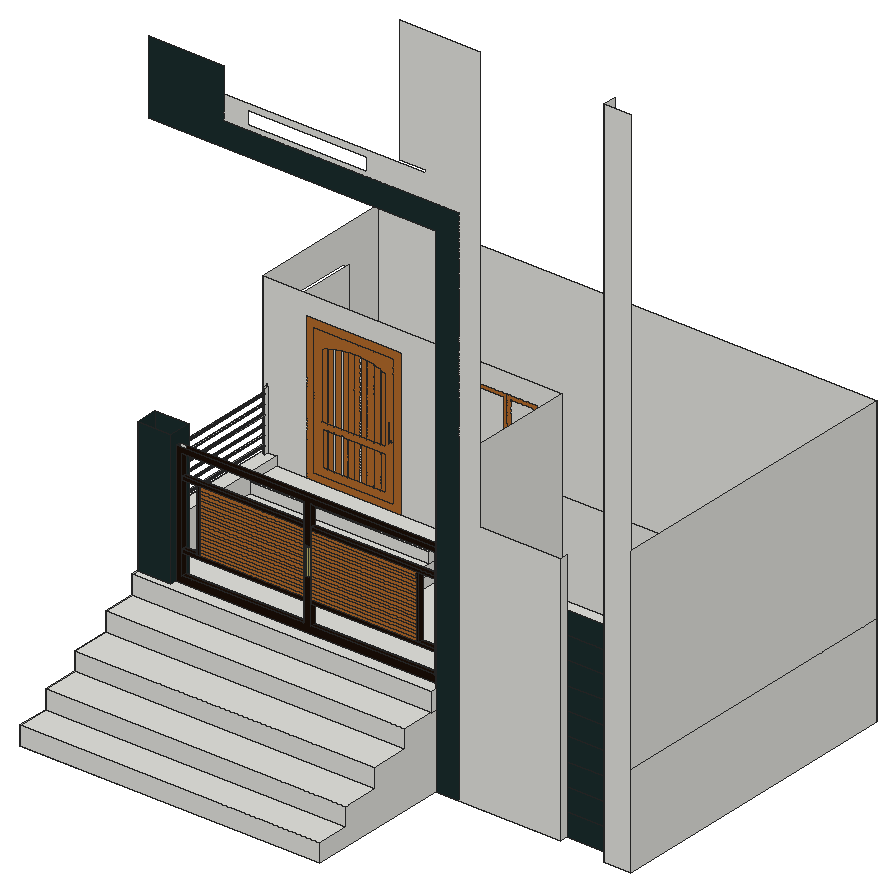
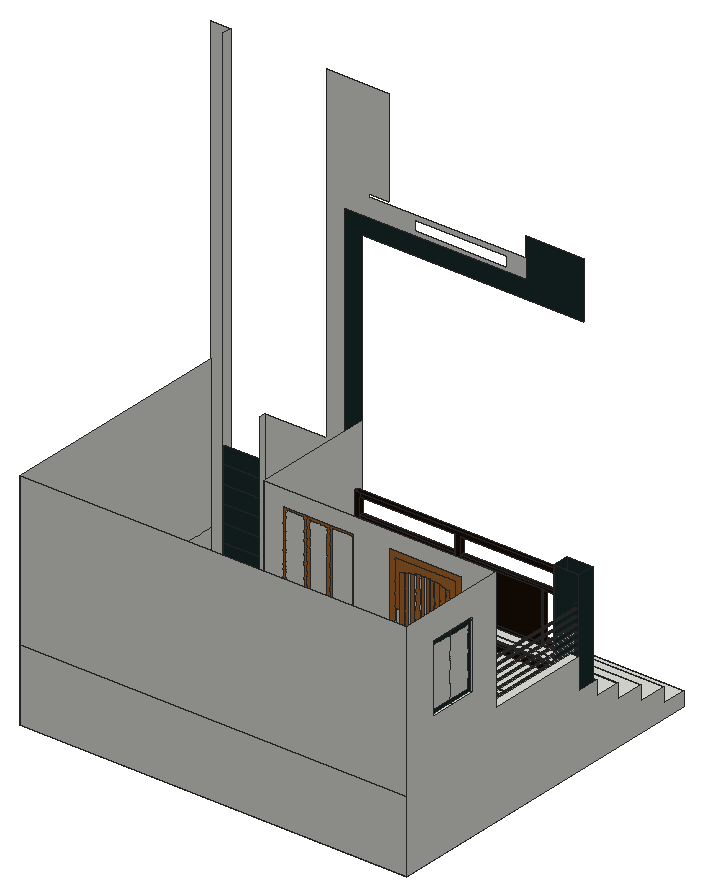
# SketchUp Ruby script. Lengths in inches.
U = 1.inch
M = Sketchup.active_model
def pt(a) = Geom::Point3d.new(a.map { |v| v * U })
def face(e, loops, mat)
  f = e.add_face(loops[0].map { |a| pt(a) })
  loops[1..].each { |l| e.add_face(l.map { |a| pt(a) }).erase! }
  f.material = f.back_material = mat if mat
  f
end
# faces: each face lists its corners as indices into pts; further lists are holes
def faces(e, pts, list, mat = nil) = list.each { |f| face(e, (f[0].is_a?(Array) ? f : [f]).map { |l| l.map { |i| pts[i] } }, mat) }
# xy, xz, yz: faces in a plane at the given z, y or x. An outline is a flat list of corners, or four numbers for a rectangle; further outlines are holes
def ring(l) = l.size == 4 ? [[l[0], l[1]], [l[2], l[1]], [l[2], l[3]], [l[0], l[3]]] : l.each_slice(2).to_a
def flat(e, list, mat, &to3) = list.each { |f| face(e, (f[0].is_a?(Array) ? f : [f]).map { |l| ring(l).map { |u, v| to3.(u, v) } }, mat) }
def xy(e, z, list, mat = nil) = flat(e, list, mat) { |x, y| [x, y, z] }
def xz(e, y, list, mat = nil) = flat(e, list, mat) { |x, z| [x, y, z] }
def yz(e, x, list, mat = nil) = flat(e, list, mat) { |y, z| [x, y, z] }
def lines(e, pts, list) = list.each { |a, b| e.add_line(pt(pts[a]), pt(pts[b])) }
# prism: a flat outline (further loops are holes) pulled along v
def prism(e, loops, v, mat = nil)
  f = face(e, loops, mat); d = Geom::Vector3d.new(v.map { |x| x * U })
  f.pushpull(f.normal.samedirection?(d) ? d.length : -d.length)
end
def box(e, o, s, mat = nil) = prism(e, [[o, [o[0] + s[0], o[1], o[2]], [o[0] + s[0], o[1] + s[1], o[2]], [o[0], o[1] + s[1], o[2]]]], [0, 0, s[2]], mat)
def at(x, y, z, deg = 0) = Geom::Transformation.translation(pt([x, y, z])) * Geom::Transformation.rotation(ORIGIN, Z_AXIS, deg.degrees)
def axes(o, x, y, z) = Geom::Transformation.new([*x, 0, *y, 0, *z, 0, *pt(o).to_a, 1])
def part(name) = M.definitions.add(name)
# library, detail: a bought-in or finely detailed component or shape, given as its bounding box
def library(name, o, s) = part(name).tap { |d| box(d.entities, o, s) }
def detail(e, o, s) = box(e.add_group.entities, o, s)
def put(e, d, t, mat = nil) = e.add_instance(d, t).tap { |i| i.material = mat if mat }
def group(e, t, mat = nil) = e.add_group.tap { |g| g.transformation = t; g.material = mat if mat }.entities
root = M.entities
M.materials.add("[0057_DarkKhaki]").color = [189, 183, 107]
M.materials.add("[0078_DarkSlateGray]").color = [27, 45, 45]
M.materials.add("[Wood Bamboo]").color = [177, 105, 43]
M.materials.add("[Wood Veneer 01]").color = [28, 16, 8]
xy(root,-50.5,[[13.625,0,13.625,274.0625,319.25,274.0625,319.25,85.75,303.01,85.75,303.01,93.625,273.68,93.625,273.68,88.9375,197.375,88.9375,197.375,0]])
xy(root,-39.2,[[13.625,0,197.375,19.5]])
xy(root,-27.9,[[13.625,19.5,197.375,42.0625]])
xy(root,-16.6,[[13.625,42.0625,197.375,65.25]])
xy(root,-5.3,[[13.625,65.25,197.375,85.75]])
xy(root,6,[[13.625,85.75,197.375,85.75,197.375,93.625,33.97,93.625,33.97,89.97,13.625,89.97],[33.97,96.69,197.375,96.69,197.375,185.5625,131.83,185.5625,131.83,141.5,22.27,141.5,22.27,103.41,33.97,103.41]])
xy(root,10.3125,[[37.47,93.625,112.35,96.69],[116.92,93.625,192.625,96.69]],"[Wood Veneer 01]")
xy(root,12.23,[[22.27,141.5,131.83,154.3125]])
xy(root,18.47,[[22.27,154.3125,131.83,165.4375]])
xy(root,22.63,[[37.47,93.625,112.35,96.69],[116.92,93.625,192.625,96.69]],"[Wood Veneer 01]")
xy(root,24.7,[[22.27,165.4375,131.83,185.5625]])
xy(root,24.71,[[46.66,93.625,48.59,96.69],[48.59,93.625,112.35,96.69],[116.92,93.625,181.16,96.69],[181.16,93.625,183.09,96.69]])
xy(root,24.71,[[37.47,93.625,46.66,96.69],[183.09,93.625,192.625,96.69]],"[Wood Veneer 01]")
xy(root,30.25,[[13.625,103.41,22.27,103.41,22.27,185.5625,17.09,185.5625,17.09,183.375,15.47,183.375,15.47,185.5625,13.625,185.5625]])
xy(root,37.79,[[113.13,92.625,114.51,93.625],[114.82,92.625,116.19,93.625]],"[0057_DarkKhaki]")
xy(root,45.65,[[16.23,103.41,16.39,183.375]])
xy(root,51.33,[[13.625,208.27,15.875,228.36],[15.875,208.27,16.1875,228.36],[13.625,228.36,15.875,248.45],[15.875,228.36,16.1875,248.45]])
xy(root,52.6,[[16.17,103.41,16.34,183.375]])
xy(root,53.42,[[113.13,92.625,114.51,93.625],[114.82,92.625,116.19,93.625]],"[0057_DarkKhaki]")
xy(root,62.69,[[46.66,93.625,48.59,96.69],[48.59,93.625,112.35,96.69],[116.92,93.625,181.16,96.69],[181.16,93.625,183.09,96.69]])
xy(root,62.69,[[37.47,93.625,46.66,96.69],[183.09,93.625,192.625,96.69]],"[Wood Veneer 01]")
xy(root,64.78,[[37.47,93.625,112.35,96.69],[116.92,93.625,192.625,96.69]],"[Wood Veneer 01]")
xz(root,0,[[13.625,-50.5,197.375,-39.2]])
xz(root,19.5,[[13.625,-39.2,197.375,-27.9]])
xz(root,42.0625,[[13.625,-27.9,197.375,-16.6]])
xz(root,65.25,[[13.625,-16.6,197.375,-5.3]])
xz(root,85.75,[[303.01,-50.5,319.25,365.8125],[13.625,-5.3,197.375,6]])
xz(root,88.9375,[[[211.43,-50.5,273.68,-50.5,273.68,104.5,224.51,104.5,224.51,365.8125,175.33,365.8125,175.33,289.25,191.33,289.25,191.33,287.4375,67.43,287.4375,67.43,272.375,211.43,272.375],[81.97,275.45,155.1,283.82]]])
xz(root,88.9375,[[197.375,-50.5,211.43,-50.5,211.43,272.375,67.43,272.375,67.43,302.875,21.25,302.875,21.25,258,197.375,258]],"[0078_DarkSlateGray]")
xz(root,89.97,[[13.625,6,33.97,88.125]],"[0078_DarkSlateGray]")
xz(root,92.625,[[113.13,37.79,114.51,53.42],[114.82,37.79,116.19,53.42]],"[0057_DarkKhaki]")
xz(root,93.625,[[273.68,-50.5,303.01,-36.62],[273.68,-36.62,303.01,-22.75],[273.68,-22.75,303.01,-8.87],[273.68,-8.87,303.01,5.01],[273.68,5.01,303.01,18.89],
  [273.68,18.89,303.01,32.76],[273.68,32.76,303.01,46.64],[273.68,46.64,303.01,60.52],[273.68,60.52,303.01,74.39]],"[0078_DarkSlateGray]")
xz(root,93.625,[[48.59,24.71,112.35,26.61],[116.92,24.71,181.16,26.61],[48.59,26.61,112.35,28.51],[116.92,26.61,181.16,28.51],[48.59,28.51,112.35,30.41],
  [116.92,28.51,181.16,30.41],[48.59,30.41,112.35,32.31],[116.92,30.41,181.16,32.31],[48.59,32.31,112.35,34.21],[116.92,32.31,181.16,34.21],
  [48.59,34.21,112.35,36.11],[116.92,34.21,181.16,36.11],[48.59,36.11,112.35,38.01],[116.92,36.11,181.16,38.01],[48.59,38.01,112.35,39.9],
  [116.92,38.01,181.16,39.9],[48.59,39.9,112.35,41.8],[116.92,39.9,181.16,41.8],[48.59,41.8,112.35,43.7],[116.92,41.8,181.16,43.7],
  [48.59,43.7,112.35,45.6],[116.92,43.7,181.16,45.6],[48.59,45.6,112.35,47.5],[116.92,45.6,181.16,47.5],[48.59,47.5,112.35,49.4],
  [116.92,47.5,181.16,49.4],[48.59,49.4,112.35,51.3],[116.92,49.4,181.16,51.3],[48.59,51.3,112.35,53.2],[116.92,51.3,181.16,53.2],
  [48.59,53.2,112.35,55.1],[116.92,53.2,181.16,55.1],[48.59,55.1,112.35,56.99],[116.92,55.1,181.16,56.99],[48.59,56.99,112.35,58.89],
  [116.92,56.99,181.16,58.89],[48.59,58.89,112.35,60.79],[116.92,58.89,181.16,60.79],[48.59,60.79,112.35,62.69],[116.92,60.79,181.16,62.69]],"[Wood Bamboo]")
xz(root,93.625,[[[33.97,6,197.375,80.73],[116.92,10.3125,192.625,77.61],[37.47,10.3125,112.35,77.61],[113.13,37.79,114.51,53.42],[114.82,37.79,116.19,53.42]],[37.47,22.63,112.35,24.71],[116.92,22.63,192.625,24.71],[46.66,24.71,48.59,62.69],[181.16,24.71,183.09,62.69],
  [37.47,62.69,112.35,64.78],[116.92,62.69,192.625,64.78]],"[Wood Veneer 01]")
xz(root,96.69,[[33.97,6,37.47,80.73]])
xz(root,96.69,[[37.47,6,192.625,10.3125],[192.625,6,197.375,80.73],[112.35,10.3125,116.92,24.71],[37.47,22.63,112.35,24.71],[116.92,22.63,192.625,24.71],
  [46.66,24.71,48.59,62.69],[48.59,24.71,112.35,62.69],[112.35,24.71,116.92,62.69],[116.92,24.71,181.16,62.69],[181.16,24.71,183.09,62.69],
  [112.35,62.69,112.35,77.61,37.47,77.61,37.47,80.73,192.625,80.73,192.625,77.61,116.92,77.61,116.92,62.69],[37.47,62.69,112.35,64.78],[116.92,62.69,192.625,64.78]],"[Wood Veneer 01]")
xz(root,103.41,[[[22.27,6,22.27,30.25,13.625,30.25,13.625,88.125,33.97,88.125,33.97,6],[15.47,66.44,17.09,68.06],[16.23,62.78,16.39,62.79,16.55,62.84,16.68,62.93,16.79,63.05,16.87,63.19,16.9,63.35,16.9,63.52,16.85,63.67,16.76,63.81,16.64,63.92,16.49,63.99,16.34,64.03,16.17,64.02,16.02,63.97,15.88,63.88,15.77,63.76,15.69,63.62,15.66,63.46,15.67,63.3,15.72,63.14,15.8,63,15.92,62.89,16.07,62.82],[16.23,57.07,16.39,57.08,16.55,57.13,16.68,57.22,16.79,57.34,16.87,57.48,16.9,57.64,16.9,57.8,16.85,57.96,16.76,58.1,16.64,58.21,16.49,58.28,16.34,58.32,16.17,58.31,16.02,58.26,15.88,58.17,15.77,58.05,15.69,57.91,15.66,57.75,15.67,57.58,15.72,57.43,15.8,57.29,15.92,57.18,16.07,57.11],[16.23,51.36,16.39,51.37,16.55,51.42,16.68,51.5,16.79,51.625,16.87,51.77,16.9,51.93,16.9,52.09,16.85,52.25,16.76,52.38,16.64,52.49,16.49,52.57,16.34,52.6,16.17,52.6,16.02,52.55,15.88,52.46,15.77,52.34,15.69,52.19,15.66,52.04,15.67,51.87,15.72,51.72,15.8,51.58,15.92,51.47,16.07,51.39],[16.23,45.65,16.39,45.65,16.55,45.7,16.68,45.79,16.79,45.91,16.87,46.06,16.9,46.22,16.9,46.38,16.85,46.53,16.76,46.67,16.64,46.78,16.49,46.86,16.34,46.89,16.17,46.88,16.02,46.84,15.88,46.75,15.77,46.63,15.69,46.48,15.66,46.32,15.67,46.16,15.72,46,15.8,45.87,15.92,45.76,16.07,45.68],[16.23,39.93,16.39,39.94,16.55,39.99,16.68,40.08,16.79,40.2,16.87,40.34,16.9,40.5,16.9,40.67,16.85,40.82,16.76,40.96,16.64,41.07,16.49,41.14,16.34,41.18,16.17,41.17,16.02,41.12,15.88,41.03,15.77,40.91,15.69,40.77,15.66,40.61,15.67,40.45,15.72,40.29,15.8,40.15,15.92,40.04,16.07,39.97],[16.23,34.22,16.39,34.23,16.55,34.28,16.68,34.37,16.79,34.49,16.87,34.63,16.9,34.79,16.9,34.95,16.85,35.11,16.76,35.25,16.64,35.36,16.49,35.43,16.34,35.47,16.17,35.46,16.02,35.41,15.88,35.32,15.77,35.2,15.69,35.06,15.66,34.9,15.67,34.73,15.72,34.58,15.8,34.44,15.92,34.33,16.07,34.26]]],"[0078_DarkSlateGray]")
xz(root,141.5,[[22.27,6,131.83,12.23]])
xz(root,154.3125,[[22.27,12.23,131.83,18.47]])
xz(root,165.4375,[[22.27,18.47,131.83,24.7]])
xz(root,183.375,[[[15.47,30.25,17.09,66.44],[16.23,62.78,16.07,62.82,15.92,62.89,15.8,63,15.72,63.14,15.67,63.3,15.66,63.46,15.69,63.62,15.77,63.76,15.88,63.88,16.02,63.97,16.17,64.02,16.34,64.03,16.49,63.99,16.64,63.92,16.76,63.81,16.85,63.67,16.9,63.52,16.9,63.35,16.87,63.19,16.79,63.05,16.68,62.93,16.55,62.84,16.39,62.79],[16.23,57.07,16.07,57.11,15.92,57.18,15.8,57.29,15.72,57.43,15.67,57.58,15.66,57.75,15.69,57.91,15.77,58.05,15.88,58.17,16.02,58.26,16.17,58.31,16.34,58.32,16.49,58.28,16.64,58.21,16.76,58.1,16.85,57.96,16.9,57.8,16.9,57.64,16.87,57.48,16.79,57.34,16.68,57.22,16.55,57.13,16.39,57.08],[16.23,51.36,16.07,51.39,15.92,51.47,15.8,51.58,15.72,51.72,15.67,51.87,15.66,52.04,15.69,52.19,15.77,52.34,15.88,52.46,16.02,52.55,16.17,52.6,16.34,52.6,16.49,52.57,16.64,52.49,16.76,52.38,16.85,52.25,16.9,52.09,16.9,51.93,16.87,51.77,16.79,51.625,16.68,51.5,16.55,51.42,16.39,51.37],[16.23,45.65,16.07,45.68,15.92,45.76,15.8,45.87,15.72,46,15.67,46.16,15.66,46.32,15.69,46.48,15.77,46.63,15.88,46.75,16.02,46.84,16.17,46.88,16.34,46.89,16.49,46.86,16.64,46.78,16.76,46.67,16.85,46.53,16.9,46.38,16.9,46.22,16.87,46.06,16.79,45.91,16.68,45.79,16.55,45.7,16.39,45.65],[16.23,39.93,16.07,39.97,15.92,40.04,15.8,40.15,15.72,40.29,15.67,40.45,15.66,40.61,15.69,40.77,15.77,40.91,15.88,41.03,16.02,41.12,16.17,41.17,16.34,41.18,16.49,41.14,16.64,41.07,16.76,40.96,16.85,40.82,16.9,40.67,16.9,40.5,16.87,40.34,16.79,40.2,16.68,40.08,16.55,39.99,16.39,39.94],[16.23,34.22,16.07,34.26,15.92,34.33,15.8,34.44,15.72,34.58,15.67,34.73,15.66,34.9,15.69,35.06,15.77,35.2,15.88,35.32,16.02,35.41,16.17,35.46,16.34,35.47,16.49,35.43,16.64,35.36,16.76,35.25,16.85,35.11,16.9,34.95,16.9,34.79,16.87,34.63,16.79,34.49,16.68,34.37,16.55,34.28,16.39,34.23]]])
xz(root,185.5625,[[[131.83,6,197.375,6,197.375,126,13.625,126,13.625,30.25,15.47,30.25,15.47,68.06,17.09,68.06,17.09,30.25,22.27,30.25,22.27,24.7,40.86,24.7,40.86,113.45,98.43,113.45,98.43,24.7,131.83,24.7],[125.82,49.72,182.38,113.9]],[53.48,33.69,53.98,55.19],[57.7,33.69,58.2,55.19],[62.14,33.69,62.64,55.19],[65.83,33.69,66.33,55.19],
  [69.48,33.69,69.98,55.19],[73.23,33.69,73.73,55.19],[77.42,33.69,77.92,55.19],[81.95,33.69,82.45,55.19],[85.98,33.69,86.48,55.19],
  [127.9375,51.84,142.55,111.78],[147.04,52.08,161.16,111.54],[165.89,52.08,180.01,111.54],[53.48,58.65,53.98,58.65,53.96,100.31,53.96,100.46,53.46,100.31],[57.7,58.65,58.2,58.65,58.18,100.23,58.18,101.61,57.68,101.49,57.68,100.31],
  [62.14,58.65,62.64,58.65,62.62,100.23,62.62,102.44,62.12,102.36,62.12,100.31],[65.83,58.65,66.33,58.65,66.3,100.23,66.3,102.84,65.8,102.79,65.8,100.31],[69.48,58.65,69.98,58.65,69.96,100.23,69.96,102.96,69.86,102.96,69.46,102.95,69.46,100.31],[73.23,58.65,73.73,58.65,73.71,100.23,73.71,102.81,73.2,102.86,73.21,100.31],[77.42,58.65,77.92,58.65,77.9,100.23,77.9,102.3125,77.4,102.39,77.4,100.31],
  [81.95,58.65,82.45,58.65,82.43,100.23,82.43,101.4,81.93,101.52,81.93,100.31],[85.98,58.65,86.48,58.65,86.46,100.23,86.26,100.31,85.96,100.4,85.96,100.31],[90.46,60.66,91.96,72.78],[92.99,62.56,93.14,62.58,93.27,62.63,93.39,62.72,93.48,62.84,93.54,62.97,93.55,63.12,93.54,63.27,93.48,63.4,93.39,63.52,93.27,63.61,93.14,63.66,92.99,63.68,92.85,63.66,92.71,63.61,92.59,63.52,92.51,63.4,92.45,63.27,92.43,63.12,92.45,62.97,92.51,62.84,92.59,62.72,92.71,62.63,92.85,62.58]])
xz(root,185.5625,[[[40.86,24.7,98.43,113.45],[45.42,29.26,93.87,108.89]],[[45.42,29.26,93.87,108.89],[50.33,58.65,50.33,99.15,53.46,100.31,53.96,100.46,56.66,101.26,57.68,101.49,58.18,101.61,59.91,102,62.12,102.36,62.62,102.44,63.2,102.54,65.8,102.79,66.3,102.84,66.53,102.86,69.46,102.95,69.86,102.96,69.96,102.96,73.2,102.86,73.71,102.81,76.52,102.54,77.4,102.39,77.9,102.3125,79.8125,102,81.93,101.52,82.43,101.4,83.0625,101.26,85.96,100.4,86.26,100.31,86.46,100.23,89.39,99.15,89.39,58.65],[50.375,33.69,89.4375,55.19],[90.46,60.66,91.96,72.78],[92.99,62.56,92.85,62.58,92.71,62.63,92.59,62.72,92.51,62.84,92.45,62.97,92.43,63.12,92.45,63.27,92.51,63.4,92.59,63.52,92.71,63.61,92.85,63.66,92.99,63.68,93.14,63.66,93.27,63.61,93.39,63.52,93.48,63.4,93.54,63.27,93.55,63.12,93.54,62.97,93.48,62.84,93.39,62.72,93.27,62.63,93.14,62.58]],[50.375,33.69,53.48,55.19],[53.98,33.69,57.7,55.19],[58.2,33.69,62.14,55.19],
  [62.64,33.69,65.83,55.19],[66.33,33.69,69.48,55.19],[69.98,33.69,73.23,55.19],[73.73,33.69,77.42,55.19],[77.92,33.69,81.95,55.19],
  [82.45,33.69,85.98,55.19],[86.48,33.69,89.4375,55.19],[[125.82,49.72,144.67,113.9],[127.9375,51.84,142.55,111.78]],[[144.67,49.72,163.53,113.9],[147.04,52.08,161.16,111.54]],[[163.53,49.72,182.38,113.9],[165.89,52.08,180.01,111.54]],
  [50.33,58.65,53.48,58.65,53.46,100.31,50.33,99.15],[53.98,58.65,57.7,58.65,57.68,100.31,57.68,101.49,56.66,101.26,53.96,100.46,53.96,100.31],[58.2,58.65,62.14,58.65,62.12,100.31,62.12,102.36,59.91,102,58.18,101.61,58.18,100.23],[62.64,58.65,65.83,58.65,65.8,100.31,65.8,102.79,63.2,102.54,62.62,102.44,62.62,100.23],[66.33,58.65,69.48,58.65,69.46,100.31,69.46,102.95,66.53,102.86,66.3,102.84,66.3,100.23],
  [69.98,58.65,73.23,58.65,73.21,100.31,73.2,102.86,69.96,102.96,69.96,100.23],[73.73,58.65,77.42,58.65,77.4,100.31,77.4,102.39,76.52,102.54,73.71,102.81,73.71,100.23],[77.92,58.65,81.95,58.65,81.93,100.31,81.93,101.52,79.8125,102,77.9,102.3125,77.9,100.23],[82.45,58.65,85.98,58.65,85.96,100.31,85.96,100.4,83.0625,101.26,82.43,101.4,82.43,100.23],[86.48,58.65,89.39,58.65,89.39,99.15,86.46,100.23]],"[Wood Bamboo]")
xz(root,208.27,[[13.625,51.33,15.875,101.9],[15.875,51.33,16.1875,101.9]])
xz(root,248.45,[[13.625,51.33,15.875,101.9],[15.875,51.33,16.1875,101.9]])
xz(root,274.0625,[[13.625,-50.5,319.25,6],[13.625,6,319.25,126]])
yz(root,13.625,[[[0,-50.5,0,-39.2,19.5,-39.2,19.5,-27.9,42.0625,-27.9,42.0625,-16.6,65.25,-16.6,65.25,-5.3,85.75,-5.3,85.75,6,103.41,6,103.41,30.25,185.5625,30.25,185.5625,126,274.0625,126,274.0625,-50.5],[208.27,51.33,248.45,105.36]]])
yz(root,13.625,[[89.97,6,103.41,88.125]],"[0078_DarkSlateGray]")
yz(root,15.47,[[183.375,30.25,185.5625,66.44]])
yz(root,15.875,[[210.84,53.91,228.36,99.32],[228.36,53.91,245.875,99.32]])
yz(root,15.875,[[208.27,51.33,208.27,101.9,228.36,101.9,228.36,99.32,210.84,99.32,210.84,53.91,228.36,53.91,228.36,51.33],[228.36,51.33,228.36,53.91,245.875,53.91,245.875,99.32,228.36,99.32,228.36,101.9,248.45,101.9,248.45,51.33]],"[0078_DarkSlateGray]")
yz(root,16.1875,[[208.27,51.33,248.45,105.36]])
yz(root,16.9,[[103.41,34.79,183.375,34.95],[103.41,40.5,183.375,40.67],[103.41,46.22,183.375,46.38],[103.41,51.93,183.375,52.09],[103.41,57.64,183.375,57.8],
  [103.41,63.35,183.375,63.52]])
yz(root,17.09,[[183.375,30.25,185.5625,66.44]])
yz(root,22.27,[[103.41,6,141.5,6,141.5,12.23,154.3125,12.23,154.3125,18.47,165.4375,18.47,165.4375,24.7,185.5625,24.7,185.5625,30.25,103.41,30.25]])
yz(root,33.97,[[89.97,6,93.625,6,93.625,80.73,96.69,80.73,96.69,6,103.41,6,103.41,88.125,89.97,88.125]],"[0078_DarkSlateGray]")
yz(root,37.47,[[93.625,22.63,96.69,24.71],[93.625,62.69,96.69,64.78]])
yz(root,37.47,[[93.625,10.3125,96.69,22.63],[93.625,24.71,96.69,62.69],[93.625,64.78,96.69,77.61]],"[Wood Veneer 01]")
yz(root,46.66,[[93.625,24.71,96.69,62.69]],"[Wood Veneer 01]")
yz(root,48.59,[[93.625,24.71,96.69,62.69]])
yz(root,112.35,[[93.625,22.63,96.69,24.71],[93.625,24.71,96.69,62.69],[93.625,62.69,96.69,64.78]])
yz(root,112.35,[[93.625,10.3125,96.69,22.63],[93.625,64.78,96.69,77.61]],"[Wood Veneer 01]")
yz(root,113.13,[[92.625,37.79,93.625,53.42]],"[0057_DarkKhaki]")
yz(root,114.51,[[92.625,37.79,93.625,53.42]],"[0057_DarkKhaki]")
yz(root,114.82,[[92.625,37.79,93.625,53.42]],"[0057_DarkKhaki]")
yz(root,116.19,[[92.625,37.79,93.625,53.42]],"[0057_DarkKhaki]")
yz(root,116.92,[[93.625,22.63,96.69,24.71],[93.625,24.71,96.69,62.69],[93.625,62.69,96.69,64.78]])
yz(root,116.92,[[93.625,10.3125,96.69,22.63],[93.625,64.78,96.69,77.61]],"[Wood Veneer 01]")
yz(root,131.83,[[141.5,6,185.5625,12.23],[154.3125,12.23,185.5625,18.47],[165.4375,18.47,185.5625,24.7]])
yz(root,183.09,[[93.625,24.71,96.69,62.69]],"[Wood Veneer 01]")
yz(root,192.625,[[93.625,22.63,96.69,24.71],[93.625,62.69,96.69,64.78]])
yz(root,192.625,[[93.625,10.3125,96.69,22.63],[93.625,24.71,96.69,62.69],[93.625,64.78,96.69,77.61]],"[Wood Veneer 01]")
yz(root,197.375,[[0,-50.5,88.9375,-50.5,88.9375,-5.3,65.25,-5.3,65.25,-16.6,42.0625,-16.6,42.0625,-27.9,19.5,-27.9,19.5,-39.2,0,-39.2],[85.75,-5.3,88.9375,6],[88.9375,6,88.9375,126,185.5625,126,185.5625,6,96.69,6,96.69,80.73,93.625,80.73,93.625,6]])
yz(root,273.68,[[88.9375,-50.5,93.625,104.5]])
yz(root,303.01,[[85.75,-50.5,93.625,365.8125]])
yz(root,319.25,[[85.75,-50.5,274.0625,6],[85.75,6,274.0625,126]])
p = [[16.07,183.375,34.26],[16.23,183.375,34.22],[16.23,103.41,34.22],[16.07,103.41,34.26],[16.39,183.375,34.23],[16.39,103.41,34.23],
  [16.55,183.375,34.28],[16.55,103.41,34.28],[15.8,183.375,34.44],[15.92,183.375,34.33],[15.92,103.41,34.33],[15.8,103.41,34.44],
  [16.68,183.375,34.37],[16.68,103.41,34.37],[15.72,183.375,34.58],[15.72,103.41,34.58],[16.79,183.375,34.49],[16.79,103.41,34.49],
  [16.87,183.375,34.63],[16.87,103.41,34.63],[15.67,183.375,34.73],[15.67,103.41,34.73],[16.9,183.375,34.79],[16.9,103.41,34.79],
  [15.66,183.375,34.9],[15.66,103.41,34.9],[15.69,183.375,35.06],[15.69,103.41,35.06],[16.9,183.375,34.95],[16.85,183.375,35.11],
  [16.85,103.41,35.11],[16.9,103.41,34.95],[15.77,183.375,35.2],[15.77,103.41,35.2],[16.76,183.375,35.25],[16.76,103.41,35.25],
  [15.88,183.375,35.32],[15.88,103.41,35.32],[16.64,183.375,35.36],[16.64,103.41,35.36],[16.02,183.375,35.41],[16.02,103.41,35.41],
  [16.17,183.375,35.46],[16.17,103.41,35.46],[16.49,183.375,35.43],[16.34,183.375,35.47],[16.34,103.41,35.47],[16.49,103.41,35.43],
  [16.07,183.375,39.97],[16.23,183.375,39.93],[16.23,103.41,39.93],[16.07,103.41,39.97],[16.39,183.375,39.94],[16.39,103.41,39.94],
  [16.55,183.375,39.99],[16.55,103.41,39.99],[15.8,183.375,40.15],[15.92,183.375,40.04],[15.92,103.41,40.04],[15.8,103.41,40.15],
  [16.68,183.375,40.08],[16.68,103.41,40.08],[16.79,183.375,40.2],[16.79,103.41,40.2],[15.72,183.375,40.29],[15.72,103.41,40.29],
  [16.87,183.375,40.34],[16.87,103.41,40.34],[15.67,183.375,40.45],[15.67,103.41,40.45],[16.9,183.375,40.5],[16.9,103.41,40.5],
  [15.66,183.375,40.61],[15.66,103.41,40.61],[15.69,183.375,40.77],[15.69,103.41,40.77],[16.9,183.375,40.67],[16.85,183.375,40.82],
  [16.85,103.41,40.82],[16.9,103.41,40.67],[15.77,183.375,40.91],[15.77,103.41,40.91],[16.76,183.375,40.96],[16.76,103.41,40.96],
  [15.88,183.375,41.03],[15.88,103.41,41.03],[16.02,183.375,41.12],[16.02,103.41,41.12],[16.64,183.375,41.07],[16.64,103.41,41.07],
  [16.17,183.375,41.17],[16.17,103.41,41.17],[16.49,183.375,41.14],[16.34,183.375,41.18],[16.34,103.41,41.18],[16.49,103.41,41.14],
  [16.07,183.375,45.68],[16.23,183.375,45.65],[16.23,103.41,45.65],[16.07,103.41,45.68],[15.92,183.375,45.76],[15.92,103.41,45.76],
  [16.39,183.375,45.65],[16.55,183.375,45.7],[16.55,103.41,45.7],[16.39,103.41,45.65],[16.68,183.375,45.79],[16.68,103.41,45.79],
  [15.8,183.375,45.87],[15.8,103.41,45.87],[16.79,183.375,45.91],[16.79,103.41,45.91],[15.72,183.375,46],[15.72,103.41,46],
  [16.87,183.375,46.06],[16.87,103.41,46.06],[15.67,183.375,46.16],[15.67,103.41,46.16],[16.9,183.375,46.22],[16.9,103.41,46.22],
  [15.66,183.375,46.32],[15.66,103.41,46.32],[15.69,183.375,46.48],[15.69,103.41,46.48],[16.9,183.375,46.38],[16.85,183.375,46.53],
  [16.85,103.41,46.53],[16.9,103.41,46.38],[15.77,183.375,46.63],[15.77,103.41,46.63],[16.76,183.375,46.67],[16.76,103.41,46.67],
  [15.88,183.375,46.75],[15.88,103.41,46.75],[16.02,183.375,46.84],[16.02,103.41,46.84],[16.64,183.375,46.78],[16.64,103.41,46.78],
  [16.17,183.375,46.88],[16.17,103.41,46.88],[16.49,183.375,46.86],[16.49,103.41,46.86],[16.34,183.375,46.89],[16.34,103.41,46.89],
  [15.92,183.375,51.47],[16.07,183.375,51.39],[16.07,103.41,51.39],[15.92,103.41,51.47],[16.23,183.375,51.36],[16.23,103.41,51.36],
  [16.39,183.375,51.37],[16.39,103.41,51.37],[16.55,183.375,51.42],[16.55,103.41,51.42],[16.68,183.375,51.5],[16.68,103.41,51.5],
  [15.8,183.375,51.58],[15.8,103.41,51.58],[16.79,183.375,51.625],[16.79,103.41,51.625],[15.72,183.375,51.72],[15.72,103.41,51.72],
  [16.87,183.375,51.77],[16.87,103.41,51.77],[15.67,183.375,51.87],[15.67,103.41,51.87],[16.9,183.375,51.93],[16.9,103.41,51.93],
  [15.66,183.375,52.04],[15.66,103.41,52.04],[15.69,183.375,52.19],[15.69,103.41,52.19],[16.9,183.375,52.09],[16.85,183.375,52.25],
  [16.85,103.41,52.25],[16.9,103.41,52.09],[15.77,183.375,52.34],[15.77,103.41,52.34],[16.76,183.375,52.38],[16.76,103.41,52.38],
  [15.88,183.375,52.46],[15.88,103.41,52.46],[16.64,183.375,52.49],[16.64,103.41,52.49],[16.02,183.375,52.55],[16.02,103.41,52.55],
  [16.17,183.375,52.6],[16.17,103.41,52.6],[16.49,183.375,52.57],[16.49,103.41,52.57],[16.34,183.375,52.6],[16.34,103.41,52.6],
  [15.92,183.375,57.18],[16.07,183.375,57.11],[16.07,103.41,57.11],[15.92,103.41,57.18],[16.23,183.375,57.07],[16.23,103.41,57.07],
  [16.39,183.375,57.08],[16.39,103.41,57.08],[16.55,183.375,57.13],[16.55,103.41,57.13],[16.68,183.375,57.22],[16.68,103.41,57.22],
  [15.8,183.375,57.29],[15.8,103.41,57.29],[16.79,183.375,57.34],[16.79,103.41,57.34],[15.72,183.375,57.43],[15.72,103.41,57.43],
  [16.87,183.375,57.48],[16.87,103.41,57.48],[15.67,183.375,57.58],[15.67,103.41,57.58],[16.9,183.375,57.64],[16.9,103.41,57.64],
  [15.66,183.375,57.75],[15.66,103.41,57.75],[15.69,183.375,57.91],[15.69,103.41,57.91],[16.9,183.375,57.8],[16.85,183.375,57.96],
  [16.85,103.41,57.96],[16.9,103.41,57.8],[15.77,183.375,58.05],[15.77,103.41,58.05],[16.76,183.375,58.1],[16.76,103.41,58.1],
  [15.88,183.375,58.17],[15.88,103.41,58.17],[16.64,183.375,58.21],[16.64,103.41,58.21],[16.02,183.375,58.26],[16.02,103.41,58.26],
  [16.49,183.375,58.28],[16.49,103.41,58.28],[16.17,183.375,58.31],[16.17,103.41,58.31],[16.34,183.375,58.32],[16.34,103.41,58.32],
  [15.92,183.375,62.89],[16.07,183.375,62.82],[16.07,103.41,62.82],[15.92,103.41,62.89],[16.23,183.375,62.78],[16.23,103.41,62.78],
  [16.39,183.375,62.79],[16.39,103.41,62.79],[16.55,183.375,62.84],[16.55,103.41,62.84],[16.68,183.375,62.93],[16.68,103.41,62.93],
  [15.8,183.375,63],[15.8,103.41,63],[16.79,183.375,63.05],[16.79,103.41,63.05],[15.72,183.375,63.14],[15.72,103.41,63.14],
  [16.87,183.375,63.19],[16.87,103.41,63.19],[15.67,183.375,63.3],[15.67,103.41,63.3],[16.9,183.375,63.35],[16.9,103.41,63.35],
  [15.66,183.375,63.46],[15.66,103.41,63.46],[15.69,183.375,63.62],[15.69,103.41,63.62],[16.9,183.375,63.52],[16.85,183.375,63.67],
  [16.85,103.41,63.67],[16.9,103.41,63.52],[15.77,183.375,63.76],[15.77,103.41,63.76],[16.76,183.375,63.81],[16.76,103.41,63.81],
  [15.88,183.375,63.88],[15.88,103.41,63.88],[16.64,183.375,63.92],[16.64,103.41,63.92],[16.02,183.375,63.97],[16.02,103.41,63.97],
  [16.49,183.375,63.99],[16.49,103.41,63.99],[16.17,183.375,64.02],[16.17,103.41,64.02],[16.34,183.375,64.03],[16.34,103.41,64.03]]
faces(root,p,[[0,1,2,3],[1,4,5,2],[4,6,7,5],[8,9,10,11],[9,0,3,10],[6,12,13,7],[14,8,11,15],[12,16,17,13],
  [16,18,19,17],[20,14,15,21],[18,22,23,19],[24,20,21,25],[26,24,25,27],[28,29,30,31],[32,26,27,33],[29,34,35,30],
  [36,32,33,37],[34,38,39,35],[40,36,37,41],[42,40,41,43],[44,45,46,47],[38,44,47,39],[45,42,43,46],[48,49,50,51],
  [49,52,53,50],[52,54,55,53],[56,57,58,59],[57,48,51,58],[54,60,61,55],[60,62,63,61],[64,56,59,65],[62,66,67,63],
  [68,64,65,69],[66,70,71,67],[72,68,69,73],[74,72,73,75],[76,77,78,79],[80,74,75,81],[77,82,83,78],[84,80,81,85],
  [86,84,85,87],[82,88,89,83],[90,86,87,91],[92,93,94,95],[88,92,95,89],[93,90,91,94],[96,97,98,99],[100,96,99,101],
  [102,103,104,105],[103,106,107,104],[108,100,101,109],[106,110,111,107],[112,108,109,113],[110,114,115,111],[116,112,113,117],[114,118,119,115],
  [120,116,117,121],[122,120,121,123],[124,125,126,127],[128,122,123,129],[125,130,131,126],[132,128,129,133],[134,132,133,135],[130,136,137,131],
  [138,134,135,139],[136,140,141,137],[142,138,139,143],[140,142,143,141],[144,145,146,147],[145,148,149,146],[148,150,151,149],[150,152,153,151],
  [152,154,155,153],[156,144,147,157],[154,158,159,155],[160,156,157,161],[158,162,163,159],[164,160,161,165],[162,166,167,163],[168,164,165,169],
  [170,168,169,171],[172,173,174,175],[176,170,171,177],[173,178,179,174],[180,176,177,181],[178,182,183,179],[184,180,181,185],[186,184,185,187],
  [182,188,189,183],[188,190,191,189],[192,193,194,195],[193,196,197,194],[196,198,199,197],[198,200,201,199],[200,202,203,201],[204,192,195,205],
  [202,206,207,203],[208,204,205,209],[206,210,211,207],[212,208,209,213],[210,214,215,211],[216,212,213,217],[218,216,217,219],[220,221,222,223],
  [224,218,219,225],[221,226,227,222],[228,224,225,229],[226,230,231,227],[232,228,229,233],[230,234,235,231],[236,232,233,237],[238,236,237,239],
  [234,238,239,235],[240,241,242,243],[241,244,245,242],[244,246,247,245],[246,248,249,247],[248,250,251,249],[252,240,243,253],[250,254,255,251],
  [256,252,253,257],[254,258,259,255],[260,256,257,261],[258,262,263,259],[264,260,261,265],[266,264,265,267],[268,269,270,271],[272,266,267,273],
  [269,274,275,270],[276,272,273,277],[274,278,279,275],[280,276,277,281],[278,282,283,279],[284,280,281,285],[286,284,285,287],[282,286,287,283]])
